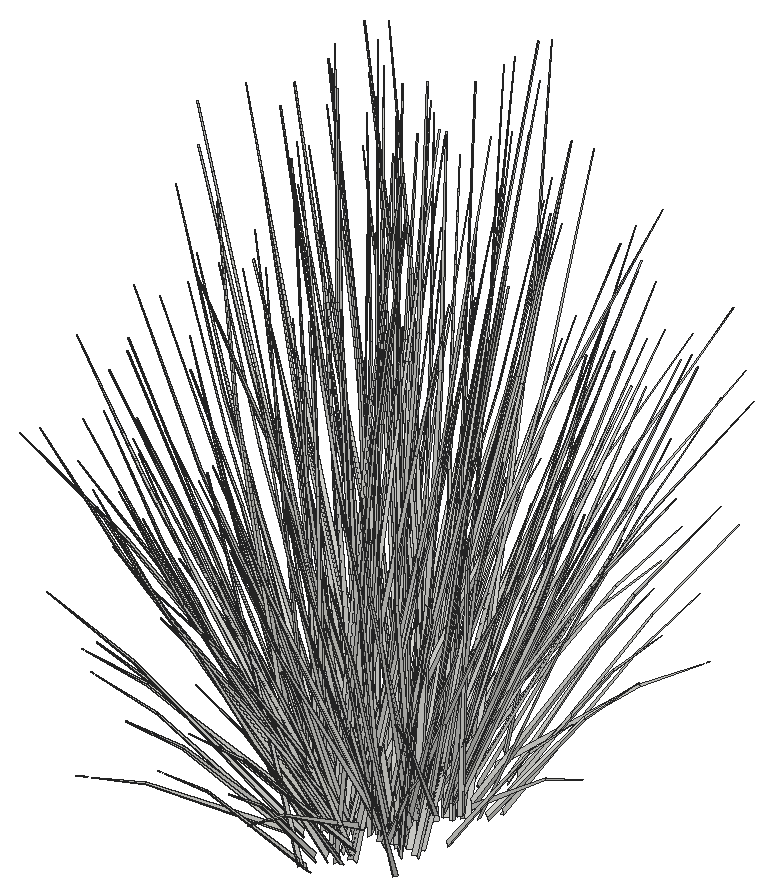
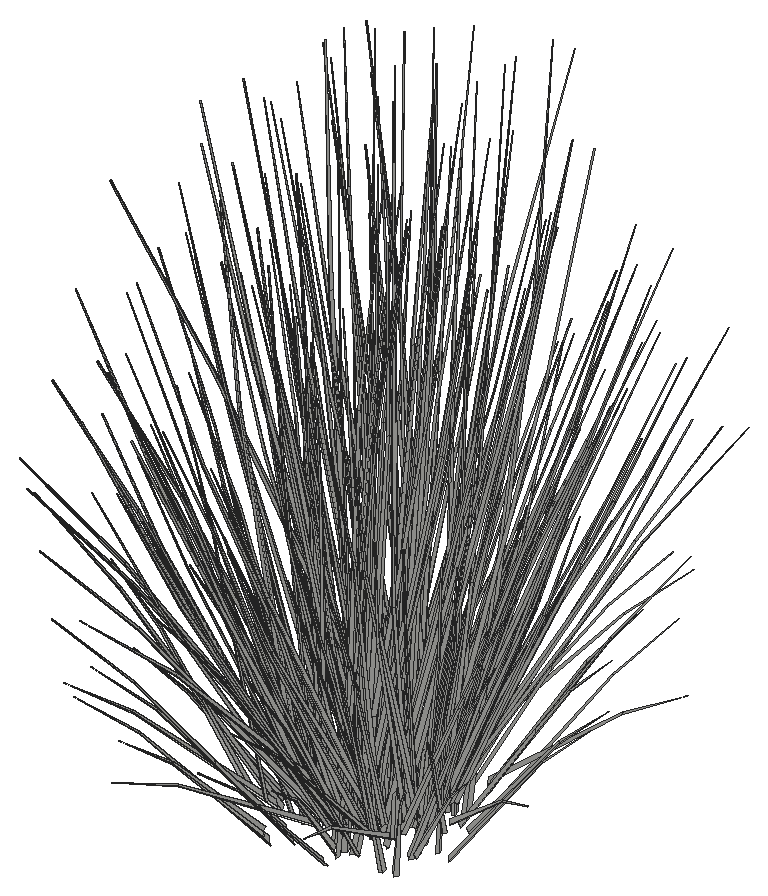
# SketchUp Ruby script. Lengths in inches.
U = 1.inch
M = Sketchup.active_model
def pt(a) = Geom::Point3d.new(a.map { |v| v * U })
def face(e, loops, mat)
  f = e.add_face(loops[0].map { |a| pt(a) })
  loops[1..].each { |l| e.add_face(l.map { |a| pt(a) }).erase! }
  f.material = f.back_material = mat if mat
  f
end
# faces: each face lists its corners as indices into pts; further lists are holes
def faces(e, pts, list, mat = nil) = list.each { |f| face(e, (f[0].is_a?(Array) ? f : [f]).map { |l| l.map { |i| pts[i] } }, mat) }
# xy, xz, yz: faces in a plane at the given z, y or x. An outline is a flat list of corners, or four numbers for a rectangle; further outlines are holes
def ring(l) = l.size == 4 ? [[l[0], l[1]], [l[2], l[1]], [l[2], l[3]], [l[0], l[3]]] : l.each_slice(2).to_a
def flat(e, list, mat, &to3) = list.each { |f| face(e, (f[0].is_a?(Array) ? f : [f]).map { |l| ring(l).map { |u, v| to3.(u, v) } }, mat) }
def xy(e, z, list, mat = nil) = flat(e, list, mat) { |x, y| [x, y, z] }
def xz(e, y, list, mat = nil) = flat(e, list, mat) { |x, z| [x, y, z] }
def yz(e, x, list, mat = nil) = flat(e, list, mat) { |y, z| [x, y, z] }
def lines(e, pts, list) = list.each { |a, b| e.add_line(pt(pts[a]), pt(pts[b])) }
# prism: a flat outline (further loops are holes) pulled along v
def prism(e, loops, v, mat = nil)
  f = face(e, loops, mat); d = Geom::Vector3d.new(v.map { |x| x * U })
  f.pushpull(f.normal.samedirection?(d) ? d.length : -d.length)
end
def box(e, o, s, mat = nil) = prism(e, [[o, [o[0] + s[0], o[1], o[2]], [o[0] + s[0], o[1] + s[1], o[2]], [o[0], o[1] + s[1], o[2]]]], [0, 0, s[2]], mat)
def at(x, y, z, deg = 0) = Geom::Transformation.translation(pt([x, y, z])) * Geom::Transformation.rotation(ORIGIN, Z_AXIS, deg.degrees)
def axes(o, x, y, z) = Geom::Transformation.new([*x, 0, *y, 0, *z, 0, *pt(o).to_a, 1])
def part(name) = M.definitions.add(name)
# library, detail: a bought-in or finely detailed component or shape, given as its bounding box
def library(name, o, s) = part(name).tap { |d| box(d.entities, o, s) }
def detail(e, o, s) = box(e.add_group.entities, o, s)
def put(e, d, t, mat = nil) = e.add_instance(d, t).tap { |i| i.material = mat if mat }
def group(e, t, mat = nil) = e.add_group.tap { |g| g.transformation = t; g.material = mat if mat }.entities
root = M.entities
c1 = part("blade")
p = [[2.15,0.21,22],[0,0.17,0],[0.09,0.45,0],[2.18,0.31,22],[2.29,0.31,22],[0.38,0.45,0],
  [2.48,0.24,33],[2.49,0.24,33],[2.48,0.22,33]]
faces(c1.entities,p,[[0,1,2,3],[4,5,2,3],[6,3,4,7],[8,0,3,6]])
c2 = part("blade with seeds\#1")
put(c2.entities,c1,at(0,0,0))
put(root,c2,axes([454.15,171.57,262.65],[-1.0019,0.47479,-0.62955],[-0.36083,-1.36768,-0.16523],[-0.33927,0.05248,1.38963]))
put(root,c2,axes([455.85,167.23,262.64],[0.89455,-0.42392,-0.62393],[0.32217,1.22114,-0.16376],[0.30292,-0.04686,1.37722]))
put(root,c2,axes([453.97,167.35,262.61],[0.16018,-1.20264,-0.5621],[0.98808,0.25378,-0.14753],[0.11973,-0.3589,1.24074]))
put(root,c2,axes([456.02,171.39,262.61],[-0.16018,1.20264,-0.5621],[-0.98808,-0.25378,-0.14753],[-0.11973,0.3589,1.24074]))
put(root,c2,axes([453.12,169.49,262.61],[-0.73437,-0.77871,-0.5621],[0.66591,-0.96736,-0.14753],[-0.18319,-0.31204,1.24074]))
put(root,c2,axes([456.87,169.25,262.61],[0.73437,0.77871,-0.5621],[-0.66591,0.96736,-0.14753],[0.18319,0.31204,1.24074]))
put(root,c2,axes([452.1,165.78,262.57],[0.48852,-1.08202,-0.44759],[0.87598,0.64674,0],[0.11126,-0.24644,1.41987]))
put(root,c2,axes([458.875,167.96,262.57],[0.48852,1.08202,-0.44759],[-0.87598,0.64674,0],[0.11126,0.24644,1.41987]))
put(root,c2,axes([454.01,174.37,262.57],[-0.97703,0,-0.44759],[0,-1.29348,0],[-0.22253,0,1.41987]))
put(root,c2,axes([457.89,172.96,262.57],[-0.48852,1.08202,-0.44759],[-0.87598,-0.64674,0],[-0.11126,0.24644,1.41987]))
put(root,c2,axes([451.11,170.78,262.57],[-0.48852,-1.08202,-0.44759],[0.87598,-0.64674,0],[-0.11126,-0.24644,1.41987]))
put(root,c2,axes([455.98,164.37,262.57],[0.97703,0,-0.44759],[0,1.29348,0],[0.22253,0,1.41987]))
put(root,c2,axes([454.41,170.85,262.75],[-0.88038,-0.56093,-0.40331],[0.4237,-1.16553,0.1941],[-0.20294,0,1.29492]))
put(root,c2,axes([455.7,170.76,262.75],[-0.82007,0.69452,-0.40331],[-0.57748,-1.05199,0.1941],[-0.10147,0.22475,1.29492]))
put(root,c2,axes([454.29,167.98,262.75],[0.82007,-0.69452,-0.40331],[0.57748,1.05199,0.1941],[0.10147,-0.22475,1.29492]))
put(root,c2,axes([455.58,167.89,262.75],[0.88038,0.56093,-0.40331],[-0.4237,1.16553,0.1941],[0.20294,0,1.29492]))
put(root,c2,axes([456.29,169.28,262.75],[0.06031,1.25545,-0.40331],[-1.00118,0.11354,0.1941],[0.10147,0.22475,1.29492]))
put(root,c2,axes([451.5,170.52,262.58],[0.24175,-1.0786,-0.27926],[0.85134,0.27158,0.27926],[-0.09817,-0.21744,1.25283]))
put(root,c2,axes([455.96,164.92,262.58],[0.60959,0.80703,-0.27926],[-0.60959,0.80703,0.27926],[0.19635,0,1.25283]))
put(root,c2,axes([457.52,172.66,262.58],[-0.85134,0.27158,-0.27926],[-0.24175,-1.0786,0.27926],[-0.09817,0.21744,1.25283]))
put(root,c2,axes([458.49,168.22,262.58],[-0.24175,1.0786,-0.27926],[-0.85134,-0.27158,0.27926],[0.09817,0.21744,1.25283]))
put(root,c2,axes([452.47,166.08,262.58],[0.85134,-0.27158,-0.27926],[0.24175,1.0786,0.27926],[0.09817,-0.21744,1.25283]))
put(root,c2,axes([454.03,173.81,262.58],[-0.60959,-0.80703,-0.27926],[0.60959,-0.80703,0.27926],[-0.19635,0,1.25283]))
put(root,c2,axes([459.05,165.83,262.1],[-0.14106,-0.08423,1.5897],[-0.41543,-1.06044,-0.24285],[0.21501,-0.3215,0.27078]))
put(root,c2,axes([454.62,175.25,262.1],[0.15398,-0.02932,1.5897],[0.80412,0.59108,-0.24285],[-0.04053,0.41985,0.27078]))
put(root,c2,axes([449.4,169.97,262.1],[0.0352,0.19392,1.5897],[-0.39624,1.07238,-0.24285],[-0.33051,-0.01799,0.27078]))
put(root,c2,axes([459.02,170.78,262.1],[-0.05317,-0.18711,1.5897],[0.29263,-1.12549,-0.24285],[0.32981,-0.03291,0.27078]))
put(root,c2,axes([454.77,162.78,262.1],[-0.14833,0.06042,1.5897],[-0.86768,-0.41907,-0.24285],[-0.01248,-0.42273,0.27078]))
put(root,c2,axes([450.61,173.4375,262.1],[0.12871,0.11199,1.5897],[0.2775,1.13173,-0.24285],[-0.25244,0.2734,0.27078]))
put(root,c2,axes([458.93,175.57,262.1],[0.09761,-0.15508,1.5897],[0.90442,-0.26295,-0.24285],[0.19286,0.3437,0.27078]))
put(root,c2,axes([451.09,165.22,262.1],[-0.07697,0.17304,1.5897],[-0.85991,0.44448,-0.24285],[-0.23336,-0.29985,0.27078]))
put(root,c2,axes([453.25,171.66,262.19],[0.39117,1.13797,1.16227],[-1.12236,0.3622,0.45161],[0.01867,-0.69878,1.32195]))
put(root,c2,axes([457.125,168,262.72],[-0.33151,-1.21377,-0.17307],[0.95493,-0.4265,0.00007],[-0.03664,-0.13398,1.56765]))
put(root,c2,axes([456.02,168.4,263.16],[1.11485,-0.13472,-0.26229],[0.06741,1.40314,-0.45076],[0.1485,0.24708,1.43974]))
put(root,c2,axes([454.85,167.75,263.16],[0.46619,-1.302,-0.26229],[0.98396,0.62692,-0.45076],[0.24158,-0.04092,1.43974]))
put(root,c2,axes([455.14,170.99,263.16],[-0.46619,1.302,-0.26229],[-0.98396,-0.62692,-0.45076],[-0.24158,0.04092,1.43974]))
put(root,c2,axes([453.97,170.34,263.16],[-1.11485,0.13472,-0.26229],[-0.06741,-1.40314,-0.45076],[-0.1485,-0.24708,1.43974]))
put(root,c2,axes([453.83,168.72,263.16],[-0.64866,-1.16728,-0.26229],[0.91655,-0.77622,-0.45076],[0.09308,-0.288,1.43974]))
put(root,c2,axes([456.16,170.02,263.16],[0.64866,1.16728,-0.26229],[-0.91655,0.77622,-0.45076],[-0.09308,0.288,1.43974]))
put(root,c2,axes([456.46,168.71,262.98],[-0.78639,1.12892,-0.2271],[-0.88305,-0.94994,0.49699],[0.09199,0.304,1.51643]))
put(root,c2,axes([456.17,170.66,262.95],[-1.15773,-0.30643,-0.21121],[0.20181,-1.4529,0.4622],[-0.15988,0.25387,1.41028]))
put(root,c2,axes([450.09,170.17,262.67],[0.56051,0.79893,-0.03509],[-0.61388,0.73204,-0.15911],[-0.17394,0.05154,0.52479]))
put(root,c2,axes([451.11,174.14,262.67],[0.7978,0.33351,-0.03509],[-0.24541,1.02647,-0.15911],[-0.13049,0.15585,0.52479]))
put(root,c2,axes([454.56,162.23,262.79],[-0.62476,0.71677,-0.05849],[-0.57245,-0.78502,-0.26518],[-0.0403,-0.22243,0.87466]))
put(root,c2,axes([455.38,163.59,262.54],[0.11725,0.74462,1.27635],[-0.9333,0.11852,0.07306],[-0.14126,-0.52153,0.72629]))
put(root,c2,axes([451.27,171.76,262.89],[-0.97904,0.72283,0],[-0.54599,-1.20931,-0.46523],[-0.12435,-0.27543,1.47583]))
put(root,c2,axes([458.48,172.3,262.89],[0.97904,0.72283,0],[-0.54599,1.20931,-0.46523],[-0.12435,0.27543,1.47583]))
put(root,c2,axes([458.72,166.98,262.89],[0.97904,-0.72283,0],[0.54599,1.20931,-0.46523],[0.12435,0.27543,1.47583]))
put(root,c2,axes([454.75,174.69,262.89],[0,1.44565,0],[-1.09198,0,-0.46523],[-0.24871,0,1.47583]))
put(root,c2,axes([457.27,168.77,262.82],[1.12244,-0.50265,-0.0542],[0.39331,1.43622,0],[0.0392,-0.01755,1.55211]))
put(root,c2,axes([451.51,166.43,262.9],[-0.97904,-0.72283,0],[0.54599,-1.20931,-0.46523],[0.12435,-0.27543,1.47583]))
put(root,c2,axes([455.24,164.05,262.9],[0,-1.44565,0],[1.09198,0,-0.46523],[0.24871,0,1.47583]))
put(root,c2,axes([455.51,168.45,262.82],[-0.84094,1.07538,-0.05527],[-0.84146,-1.07603,0],[-0.02937,0.03755,1.58274]))
put(root,c2,axes([455.09,168.08,262.82],[1.12994,0,-0.05082],[0,1.44565,0],[0.03551,0,1.61697]))
put(root,c2,axes([458.61,167.89,262.73],[-0.98246,0.71382,-0.04636],[-0.54599,-1.20931,0.46523],[0.09354,0.298,1.4751]))
put(root,c2,axes([455.8,164.62,262.74],[-0.00781,1.44494,-0.04486],[-1.09198,0,0.45022],[0.24858,0.04541,1.42752]))
put(root,c2,axes([454.46,173.57,262.85],[0.82143,1.07538,0.27726],[-0.81279,1.07603,-0.32897],[-0.23327,0.03755,1.48641]))
put(root,c2,axes([458.11,167.86,262.85],[0.31757,-1.44738,0.27726],[1.13512,0.3621,-0.32897],[0.14207,0.23956,1.48641]))
put(root,c2,axes([457.625,169.68,262.73],[-0.43865,1.16553,0],[-0.91144,-0.56093,0],[0,0,1.46678]))
put(root,c2,axes([457.24,169.41,262.74],[-0.84234,0.37722,0],[-0.29498,-1.07717,0],[0,0,1.39163]))
put(root,c2,axes([457.64,168.35,262.74],[0.43865,-1.16553,0],[0.91144,0.56093,0],[0,0,1.57718]))
put(root,c2,axes([454.64,168.81,262.74],[-1.1305,0,0],[0,-1.44565,0],[0,0,1.61777]))
put(root,c2,axes([454.89,167.83,262.74],[0,-1.29348,0],[1.0115,0,0],[0,0,1.60831]))
put(root,c2,axes([455.32,167.86,262.75],[0.63109,-0.80703,0],[0.63109,0.80703,0],[0,0,1.52591]))
put(root,c2,axes([455.61,170.49,262.88],[0.20585,-1.46124,0.41247],[1.16261,0.29738,0.16186],[-0.11226,0.21355,1.43206]))
put(root,c2,axes([453.92,169.49,262.88],[0.88667,0.95859,0.41247],[-0.7827,1.13884,0.16186],[-0.08849,-0.2311,1.43206]))
put(root,c2,axes([454.54,170.62,262.88],[1.09253,-0.50265,0.41247],[0.37991,1.43622,0.16186],[-0.20075,-0.01755,1.43206]))
put(root,c2,axes([454.375,168.25,262.9],[-0.20585,1.46124,0.44352],[-1.16261,-0.29738,0.17404],[0.11226,-0.21355,1.53985]))
put(root,c2,axes([456.24,168.14,263.11],[0.58702,-0.85413,0.13053],[0.66228,0.71246,-0.37274],[0.08953,0.19831,1.14258]))
put(root,c2,axes([453.54,168.61,263.11],[-0.87196,-0.22303,0.13053],[0.15136,-1.08968,-0.37274],[0.08953,-0.19831,1.14258]))
put(root,c2,axes([454.79,167.38,263.11],[-0.28493,-1.07717,0.13053],[0.81364,-0.37722,-0.37274],[0.17907,0,1.14258]))
put(root,c2,axes([456.45,170.13,263.11],[0.87196,0.22303,0.13053],[-0.15136,1.08968,-0.37274],[-0.08953,0.19831,1.14258]))
put(root,c2,axes([459.15,173.37,263.3],[-0.17302,-1.05027,0.05866],[0.69705,-0.24145,-0.77802],[0.35285,0.06658,0.69739]))
put(root,c2,axes([452.8,174.45,263.09],[0.27202,-0.22572,1.28914],[0.7394,0.52014,-0.27724],[-0.17673,0.53408,0.55117]))
put(root,c2,axes([459.89,173.62,263.09],[-0.15413,-0.36483,1.28914],[0.46474,-0.90077,-0.27724],[0.40213,0.2681,0.55117]))
put(root,c2,axes([457.71,168.33,263.09],[-0.32388,-0.0204,1.28914],[-0.36177,-0.97496,-0.27724],[0.38765,-0.30097,0.55117]))
put(root,c2,axes([450.47,167.52,263.09],[0.19776,0.32863,1.28914],[-0.34614,0.98419,-0.27724],[-0.43048,-0.18244,0.55117]))
put(root,c2,axes([452.8,164.35,263.09],[-0.02894,0.41302,1.28914],[-0.77632,0.42312,-0.27724],[-0.21961,-0.50739,0.55117]))
put(root,c2,axes([450.1,172.61,263.09],[0.31962,0.07001,1.28914],[0.26756,1.02347,-0.27724],[-0.41311,0.23924,0.55117]))
put(root,c2,axes([456.77,163.38,263.09],[-0.2403,0.27843,1.28914],[-0.79492,-0.36227,-0.27724],[0.10768,-0.56334,0.55117]))
put(root,c2,axes([456.76,176,263.09],[0.08021,-0.40179,1.28914],[0.81924,-0.25896,-0.27724],[0.15335,0.54576,0.55117]))
put(root,c2,axes([454.91,173.81,262.99],[0.97703,0,0.44759],[0,1.29348,0],[-0.22253,0,1.41987]))
put(root,c2,axes([452.02,167.06,262.99],[-0.48852,1.08202,0.44759],[-0.87598,-0.64674,0],[0.11126,-0.24644,1.41987]))
put(root,c2,axes([455.08,164.92,262.99],[-0.97703,0,0.44759],[0,-1.29348,0],[0.22253,0,1.41987]))
put(root,c2,axes([458.05,167.24,262.99],[-0.48852,-1.08202,0.44759],[0.87598,-0.64674,0],[0.11126,0.24644,1.41987]))
put(root,c2,axes([457.97,171.68,262.99],[0.48852,-1.08202,0.44759],[0.87598,0.64674,0],[-0.11126,0.24644,1.41987]))
put(root,c2,axes([454.84,170.15,262.95],[0.47355,-1.30265,0.21694],[0.98396,0.62692,0.45076],[-0.22682,0,1.44726]))
put(root,c2,axes([452.52,167.46,262.98],[0.25932,1.24233,0.15904],[-0.96507,0.30677,0.3163],[0.14061,-0.1108,1.44604]))
put(root,c2,axes([455.05,165.67,262.98],[-0.71168,0.90835,0.15904],[-0.69029,-0.91538,0.3163],[0.14534,0.10032,1.44604]))
put(root,c2,axes([452.46,171.16,262.98],[0.971,0.33398,0.15904],[-0.27478,1.22215,0.3163],[-0.00473,-0.21112,1.44604]))
put(root,c2,axes([457.53,167.58,262.98],[-0.971,-0.33398,0.15904],[0.27478,-1.22215,0.3163],[0.00473,0.21112,1.44604]))
put(root,c2,axes([457.47,171.28,262.98],[-0.25932,-1.24233,0.15904],[0.96507,-0.30677,0.3163],[-0.14061,0.1108,1.44604]))
put(root,c2,axes([454.58,167.87,263.2],[-0.88038,-0.56093,0.40331],[0.4237,-1.16553,-0.1941],[0.20294,0,1.29492]))
put(root,c2,axes([454.18,170.57,263.2],[0.06031,1.25545,0.40331],[-1.00118,0.11354,-0.1941],[-0.10147,-0.22475,1.29492]))
put(root,c2,axes([453.77,169.07,263.2],[-0.82007,0.69452,0.40331],[-0.57748,-1.05199,-0.1941],[0.10147,-0.22475,1.29492]))
put(root,c2,axes([455.4,170.87,263.2],[0.88038,0.56093,0.40331],[-0.4237,1.16553,-0.1941],[-0.20294,0,1.29492]))
put(root,c2,axes([455.81,168.16,263.2],[-0.06031,-1.25545,0.40331],[1.00118,-0.11354,-0.1941],[0.10147,0.22475,1.29492]))
put(root,c2,axes([459.29,165.91,263.16],[-0.03064,0.74138,0.9471],[-0.6508,-0.48961,0.52291],[0.23122,-0.29288,0.74292]))
put(root,c2,axes([453.61,175.79,263.25],[-0.06991,-0.73811,1.03545],[0.616,0.4682,0.76078],[-0.09241,0.36475,0.22807]))
put(root,c2,axes([458.01,166.01,263.25],[-0.28093,0.65095,1.03545],[-0.28545,-0.84053,0.76078],[0.2418,-0.22671,0.22807]))
put(root,c2,axes([458.48,176.84,263.25],[-0.44281,-0.48182,1.03545],[0.70101,-0.19012,0.76078],[0.12552,0.34819,0.22807]))
put(root,c2,axes([455.7,162.04,263.25],[0.1613,0.71432,1.03545],[-0.66662,-0.33623,0.76078],[0.04561,-0.37895,0.22807]))
put(root,c2,axes([449.59,172.96,263.25],[0.34005,-0.60308,1.03545],[0.20441,0.87829,0.76078],[-0.26134,0.18792,0.22807]))
put(root,c2,axes([460.41,172.75,263.25],[-0.58095,0.02992,1.03545],[0.41436,-0.74764,0.76078],[0.2769,0.14704,0.22807]))
put(root,c2,axes([451.375,163.88,263.25],[0.49736,0.38508,1.03545],[-0.66822,0.331,0.76078],[-0.16744,-0.31805,0.22807]))
put(root,c2,axes([448.9,168.73,263.25],[0.56973,-0.14831,1.03545],[-0.31555,0.82274,0.76078],[-0.29172,-0.08853,0.22807]))
put(root,c2,axes([454.85,167.6,263.32],[-0.91991,0.03158,1.27354],[0.23846,-1.42935,0.53923],[0.50337,0.33806,1.20213]))
put(root,c2,axes([451.39,171.51,265.24],[-0.47225,0.98582,-0.64046],[-0.82754,-0.7006,0.07729],[-0.28197,0.35717,0.906]))
put(root,c2,axes([458.64,170.43,265.24],[0.79444,-0.5518,-0.64046],[0.44274,1.13586,0.07729],[0.38385,-0.12903,0.906]))
put(root,c2,axes([452.56,173.51,265.24],[-0.02352,1.1557,-0.64046],[-0.99061,-0.07762,0.07729],[-0.10454,0.48961,0.906]))
put(root,c2,axes([453.51,165.23,265.24],[-0.77091,-0.6039,-0.64046],[0.54787,-1.05824,0.07729],[-0.27931,-0.36058,0.906]))
put(root,c2,axes([455.46,164.94,265.24],[-0.4315,-1.0159,-0.64046],[0.88824,-0.56616,0.07729],[-0.1009,-0.49086,0.906]))
put(root,c2,axes([451.94,166.72,265.24],[-0.90375,-0.03008,-0.64046],[0.0607,-1.26677,0.07729],[-0.38287,-0.13368,0.906]))
put(root,c2,axes([457.25,165.93,265.24],[0.02352,-1.1557,-0.64046],[0.99061,0.07762,0.07729],[0.10454,-0.48961,0.906]))
put(root,c2,axes([451.16,169.02,265.24],[-0.79444,0.5518,-0.64046],[-0.44274,-1.13586,0.07729],[-0.38385,0.12903,0.906]))
put(root,c2,axes([458.8,170.02,264.97],[0.24493,-1.13649,-0.46065],[0.83975,0.38955,-0.35681],[0.33809,-0.10421,0.88141]))
put(root,c2,axes([451.64,166.98,264.97],[-0.65648,0.82762,-0.46065],[-0.57493,-0.87428,-0.35681],[-0.33354,-0.12593,0.88141]))
put(root,c2,axes([451.41,171.97,264.97],[0.23225,1.14083,-0.46065],[-0.87956,0.19957,-0.35681],[-0.25205,0.30642,0.88141]))
put(root,c2,axes([455.13,164.74,264.97],[-0.88873,-0.31321,-0.46065],[0.30463,-1.07385,-0.35681],[-0.08149,-0.43235,0.88141]))
put(root,c2,axes([452.76,173.9,264.97],[0.6472,0.83949,-0.46065],[-0.68369,0.73521,-0.35681],[-0.09847,0.42653,0.88141]))
put(root,c2,axes([456.66,174.19,264.97],[0.89213,-0.297,-0.46065],[0.15606,1.12475,-0.35681],[0.23962,0.32232,0.88141]))
put(root,c2,axes([454.68,174.71,264.97],[0.88873,0.31321,-0.46065],[-0.30463,1.07385,-0.35681],[0.08149,0.43235,0.88141]))
put(root,c2,axes([451,169.43,264.97],[-0.24493,1.13649,-0.46065],[-0.83975,-0.38955,-0.35681],[-0.33809,0.10421,0.88141]))
put(root,c2,axes([453.15,165.26,264.97],[-0.89213,0.297,-0.46065],[-0.15606,-1.12475,-0.35681],[-0.23962,-0.32232,0.88141]))
put(root,c2,axes([458.4,167.48,264.97],[-0.23225,-1.14083,-0.46065],[0.87956,-0.19957,-0.35681],[0.25205,-0.30642,0.88141]))
put(root,c2,axes([454.14,172.44,263.77],[-0.14134,-0.32863,1.5962],[0.98684,-0.11332,0.12492],[0.13095,0.71181,0.57049]))
put(root,c2,axes([457.87,172.73,265.57],[0.90375,0.03008,-0.71091],[-0.0607,1.26677,0.08579],[0.38287,0.13368,1.00565]))
put(root,c2,axes([458.17,172.47,265.27],[0.65648,-0.82762,-0.51132],[0.57493,0.87428,-0.39606],[0.33354,0.12593,0.97836]))
put(root,c2,axes([459.14,173.15,263.79],[-0.50438,-0.0254,1.3914],[0.26641,-1.14247,0.19228],[0.53755,0.09899,0.65702]))
put(root,c2,axes([456.73,169.15,263.75],[0.39398,-0.99907,1.36359],[0.84877,0.97875,0.53923],[-0.50305,0.4384,1.14314]))
put(root,c2,axes([457.66,165.24,264.83],[0.61172,-0.65782,-0.31925],[0.57907,0.75112,0.41216],[0.08811,-0.38163,0.78863]))
put(root,c2,axes([454.27,175.37,264.83],[-0.27256,0.96081,-0.31925],[-0.79518,-0.28024,0.41216],[0.07291,0.38684,0.78863]))
put(root,c2,axes([456.5625,175.02,264.83],[0.13963,1.00636,-0.31925],[-0.79822,0.26574,0.41216],[0.2144,0.28839,0.78863]))
put(root,c2,axes([455.54,164.08,264.83],[0.27256,-0.96081,-0.31925],[0.79518,0.28024,0.41216],[-0.07291,-0.38684,0.78863]))
put(root,c2,axes([450.76,171.85,264.83],[-0.78697,0.17856,-0.31925],[-0.2078,-1.02074,0.41216],[-0.22552,0.27417,0.78863]))
put(root,c2,axes([458.41,173.25,264.83],[0.51441,0.78225,-0.31925],[-0.58738,0.7405,0.41216],[0.29843,0.11267,0.78863]))
put(root,c2,axes([453.24,164.43,264.83],[-0.13963,-1.00636,-0.31925],[0.79822,-0.26574,0.41216],[-0.2144,-0.28839,0.78863]))
put(root,c2,axes([459.32,170.53,264.83],[0.75135,0.34854,-0.31925],[-0.21915,1.01686,0.41216],[0.30251,-0.09324,0.78863]))
put(root,c2,axes([451.4,166.2,264.83],[-0.51441,-0.78225,-0.31925],[0.58738,-0.7405,0.41216],[-0.29843,-0.11267,0.78863]))
put(root,c2,axes([450.49,168.91,264.83],[-0.75135,-0.34854,-0.31925],[0.21915,-1.01686,0.41216],[-0.30251,0.09324,0.78863]))
put(root,c2,axes([452.15,174.21,264.83],[-0.61172,0.65782,-0.31925],[-0.57907,-0.75112,0.41216],[-0.08811,0.38163,0.78863]))
put(root,c2,axes([457.75,163.28,264.3],[-0.82131,0.22128,-0.03148],[-0.18882,-1.04586,-0.14272],[0.05207,-0.2184,0.47074]))
put(root,c2,axes([456.09,167.6,264.25],[-0.16834,0.42944,1.54493],[-0.70619,-0.88871,0.12492],[0.31858,-0.5539,0.66044]))
put(root,c2,axes([451.48,168.15,264.25],[0.33582,0.21526,1.54493],[-0.69497,0.90306,0.12492],[-0.43315,-0.40739,0.66044]))
put(root,c2,axes([454.55,166.7,264.25],[0.02213,0.47954,1.54493],[-0.95907,-0.31812,0.12492],[0.05932,-0.68338,0.66044]))
put(root,c2,axes([457.07,169.37,264.25],[-0.31369,0.26428,1.54493],[-0.26409,-1.22118,0.12492],[0.49247,-0.276,0.66044]))
put(root,c2,axes([457.23,171.53,264.25],[-0.375,0.0283,1.54493],[0.24877,-1.22643,0.12492],[0.53441,0.07586,0.66044]))
put(root,c2,axes([456.52,173.5,264.25],[-0.33582,-0.21526,1.54493],[0.69497,-0.90306,0.12492],[0.43315,0.40739,0.66044]))
put(root,c2,axes([455.13,174.75,264.25],[-0.20666,-0.40114,1.54493],[0.95496,-0.33772,0.12492],[0.21583,0.62976,0.66044]))
put(root,c2,axes([455.78,173.28,264.25],[-0.3002,-0.28876,1.54493],[0.81031,-0.72911,0.12492],[0.36902,0.50009,0.66044]))
put(root,c2,axes([450.93,172.27,264.25],[0.31369,-0.26428,1.54493],[0.26409,1.22118,0.12492],[-0.49247,0.276,0.66044]))
put(root,c2,axes([451.91,174.04,264.25],[0.16834,-0.42944,1.54493],[0.70619,0.88871,0.12492],[-0.31858,0.5539,0.66044]))
put(root,c2,axes([453.45,174.95,264.25],[-0.02213,-0.47954,1.54493],[0.95907,0.31812,0.12492],[-0.05932,0.68338,0.66044]))
put(root,c2,axes([457.73,165.99,265.29],[-0.99362,-0.0619,-0.10962],[0.02716,-1.17208,-0.60845],[0.06902,-0.45141,0.92453]))
put(root,c2,axes([453.92,174.76,265.29],[0.88471,-0.5817,-0.10962],[0.43476,1.03242,-0.60845],[0.11673,0.43507,0.92453]))
put(root,c2,axes([451.98,166.11,265.29],[-0.04841,1.27062,-0.10962],[-0.91657,-0.03473,-0.60845],[-0.353,-0.08826,0.92453]))
put(root,c2,axes([455.89,164.68,265.29],[-0.88471,0.5817,-0.10962],[-0.43476,-1.03242,-0.60845],[-0.11673,-0.43507,0.92453]))
put(root,c2,axes([458.84,170.99,265.29],[-0.45489,-1.13134,-0.10962],[0.80735,-0.55596,-0.60845],[0.34022,-0.14927,0.92453]))
put(root,c2,axes([452.08,173.46,265.29],[0.99362,0.0619,-0.10962],[-0.02716,1.17208,-0.60845],[-0.06902,0.45141,0.92453]))
put(root,c2,axes([458.81,168.3,265.29],[-0.8363,-0.68892,-0.10962],[0.4818,-0.99769,-0.60845],[0.23628,-0.3468,0.92453]))
put(root,c2,axes([456.02,174.72,265.29],[0.53874,-1.06944,-0.10962],[0.78019,0.61612,-0.60845],[0.2712,0.30214,0.92453]))
put(root,c2,axes([450.96,168.46,265.29],[0.45489,1.13134,-0.10962],[-0.80735,0.55596,-0.60845],[-0.34022,0.14927,0.92453]))
put(root,c2,axes([453.79,164.73,265.29],[-0.53874,1.06944,-0.10962],[-0.78019,-0.61612,-0.60845],[-0.2712,-0.30214,0.92453]))
put(root,c2,axes([453.875,167.52,264.79],[-0.50765,0.99901,1.24659],[-0.79039,-1.05487,0.53787],[0.47632,-0.32232,1.20495]))
put(root,c2,axes([454.8,175.98,265],[0.12685,0.18879,1.57709],[0.92682,-0.01606,-0.24942],[0.12053,0.43275,0.12648]))
put(root,c2,axes([454.5,161.53,265],[-0.14882,-0.16043,1.57709],[-0.91289,0.20534,-0.24942],[-0.17308,-0.40254,0.12648]))
put(root,c2,axes([457.13,164.97,265],[-0.01652,-0.24801,1.57709],[-0.75906,-0.68026,-0.24942],[0.1002,-0.44114,0.12648]))
put(root,c2,axes([450.53,164.96,265],[-0.19445,0.01116,1.57709],[-0.562,0.94258,-0.24942],[-0.34067,-0.14573,0.12648]))
put(root,c2,axes([458.26,175.95,265],[0.19335,0.02874,1.57709],[0.67262,-0.81555,-0.24942],[0.31807,0.21351,0.12648]))
put(root,c2,axes([460.65,171.25,265],[0.15733,-0.14655,1.57709],[0.06181,-1.18266,-0.24942],[0.34698,-0.11893,0.12648]))
put(root,c2,axes([448.85,170.26,265],[-0.13699,0.17683,1.57709],[0.08685,1.18009,-0.24942],[-0.32765,0.18834,0.12648]))
put(root,c2,axes([450.36,174.125,265],[-0.0069,0.24875,1.57709],[0.68965,0.79195,-0.24942],[-0.14092,0.42256,0.12648]))
put(root,c2,axes([450.94,175.08,265],[0.0975,-0.08571,1.59908],[0.87648,0.41319,-0.1511],[0.00634,0.41846,0.28298]))
put(root,c2,axes([448.4,171.47,265],[0.11711,0.02157,1.59908],[0.42502,1.06376,-0.1511],[-0.21726,0.31303,0.28298]))
put(root,c2,axes([459.5,169.2,265],[-0.11829,-0.00342,1.59908],[-0.52187,-0.99076,-0.1511],[0.18628,-0.34414,0.28298]))
put(root,c2,axes([455.74,178.07,265],[0.0262,-0.14755,1.59908],[0.86326,-0.45644,-0.1511],[0.22658,0.30203,0.28298]))
put(root,c2,axes([453.56,162.1,265],[-0.00742,0.151,1.59908],[-0.79509,0.62706,-0.1511],[-0.26143,-0.25182,0.28298]))
put(root,c2,axes([458.52,162.37,265],[-0.08553,0.10454,1.59908],[-0.91687,-0.22868,-0.1511],[-0.05858,-0.41178,0.28298]))
put(root,c2,axes([460.24,176.04,265],[-0.05899,-0.13116,1.59908],[0.39237,-1.08407,-0.1511],[0.32669,0.02548,0.28298]))
put(root,c2,axes([449.83,165.21,265],[0.07463,0.11741,1.59908],[-0.25178,1.15035,-0.1511],[-0.32567,0.04164,0.28298]))
put(root,c2,axes([457.82,173.34,265.62],[0.04841,-1.27062,-0.12168],[0.91657,0.03473,-0.67538],[0.353,0.08826,1.02623]))
put(root,c2,axes([450.625,171.17,265.65],[0.93666,0.77159,-0.12278],[-0.53962,1.11741,-0.68147],[-0.26463,0.38842,1.03548]))
put(root,c2,axes([450.66,168.79,265.02],[0.25543,-1.1392,0.43274],[0.83975,0.38955,0.35681],[-0.33023,0.06846,0.89544]))
put(root,c2,axes([457.66,165.49,265.02],[0.64379,0.85247,0.43274],[-0.68369,0.73521,0.35681],[0.11875,-0.39995,0.89544]))
put(root,c2,axes([455.64,164.3,265.02],[0.89085,0.32663,0.43274],[-0.30463,1.07385,0.35681],[-0.05354,-0.4223,0.89544]))
put(root,c2,axes([456.39,174.89,265.02],[-0.89921,0.28673,0.43274],[-0.15606,-1.12475,0.35681],[0.21148,0.33149,0.89544]))
put(root,c2,axes([458.21,173.25,265.02],[-0.66663,0.82326,0.43274],[-0.57493,-0.87428,0.35681],[0.31276,0.15186,0.89544]))
put(root,c2,axes([451.6,166.2,265.02],[0.66663,-0.82326,0.43274],[0.57493,0.87428,0.35681],[-0.31276,-0.15186,0.89544]))
put(root,c2,axes([454.17,175.15,265.02],[-0.89085,-0.32663,0.43274],[0.30463,-1.07385,0.35681],[0.05354,0.4223,0.89544]))
put(root,c2,axes([453.42,164.56,265.02],[0.89921,-0.28673,0.43274],[0.15606,1.12475,0.35681],[-0.21148,-0.33149,0.89544]))
put(root,c2,axes([458.94,167.82,265.02],[0.22422,1.14989,0.43274],[-0.87956,0.19957,0.35681],[0.25922,-0.27044,0.89544]))
put(root,c2,axes([450.69,171.4,265.02],[-0.62066,-0.52545,0.05797],[0.36135,-0.74826,0.45634],[-0.19899,0.24191,0.69585]))
put(root,c2,axes([459.21,170.96,265.02],[0.33205,0.8519,0.05797],[-0.60551,0.41697,0.45634],[0.26692,-0.08227,0.69585]))
put(root,c2,axes([453.59,164.34,265.02],[0.4109,-0.79368,0.05797],[0.58514,0.46209,0.45634],[-0.18917,-0.25446,0.69585]))
put(root,c2,axes([455.87,164.22,265.02],[0.66618,-0.42462,0.05797],[0.32607,0.77431,0.45634],[-0.06434,-0.34133,0.69585]))
put(root,c2,axes([451.91,173.87,265.02],[-0.74296,-0.05822,0.05797],[0.02037,-0.87906,0.45634],[-0.07774,0.33673,0.69585]))
put(root,c2,axes([451.66,165.9,265.02],[0.04552,-0.95007,0.05797],[0.68742,0.02605,0.45634],[-0.26332,-0.09941,0.69585]))
put(root,c2,axes([457.89,165.58,265.02],[0.74296,0.05822,0.05797],[-0.02037,0.87906,0.45634],[0.07774,-0.33673,0.69585]))
put(root,c2,axes([456.22,175.11,265.02],[-0.4109,0.79368,0.05797],[-0.58514,-0.46209,0.45634],[0.18917,0.25446,0.69585]))
put(root,c2,axes([450.6,168.49,265.02],[-0.33205,-0.8519,0.05797],[0.60551,-0.41697,0.45634],[-0.26692,0.08227,0.69585]))
put(root,c2,axes([453.9375,175.23,265.02],[-0.66618,0.42462,0.05797],[-0.32607,-0.77431,0.45634],[0.06434,0.34133,0.69585]))
put(root,c2,axes([459.12,168.04,265.02],[0.62066,0.52545,0.05797],[-0.36135,0.74826,0.45634],[0.19899,-0.24191,0.69585]))
put(root,c2,axes([458.15,173.55,265.02],[-0.04552,0.95007,0.05797],[-0.68742,-0.02605,0.45634],[0.26332,0.09941,0.69585]))
put(root,c2,axes([458.53,170.65,265.31],[-0.75135,-0.34854,0.31925],[0.21915,-1.01686,-0.41216],[0.30251,-0.09324,0.78863]))
put(root,c2,axes([451.28,168.8,265.31],[0.75135,0.34854,0.31925],[-0.21915,1.01686,-0.41216],[-0.30251,0.09324,0.78863]))
put(root,c2,axes([457.34,166.17,265.31],[-0.61172,0.65782,0.31925],[-0.57907,-0.75112,-0.41216],[0.08811,-0.38163,0.78863]))
put(root,c2,axes([455.625,165.09,265.31],[-0.27256,0.96081,0.31925],[-0.79518,-0.28024,-0.41216],[-0.07291,-0.38684,0.78863]))
put(root,c2,axes([452.47,173.28,265.31],[0.61172,-0.65782,0.31925],[0.57907,0.75112,-0.41216],[-0.08811,0.38163,0.78863]))
put(root,c2,axes([457.68,172.84,265.31],[-0.51441,-0.78225,0.31925],[0.58738,-0.7405,-0.41216],[0.29843,0.11267,0.78863]))
put(root,c2,axes([456.09,174.2,265.31],[-0.13963,-1.00636,0.31925],[0.79822,-0.26574,-0.41216],[0.2144,0.28839,0.78863]))
put(root,c2,axes([458.4,168.21,265.31],[-0.78697,0.17856,0.31925],[-0.2078,-1.02074,-0.41216],[0.22552,-0.27417,0.78863]))
put(root,c2,axes([453.72,165.25,265.31],[0.13963,1.00636,0.31925],[-0.79822,0.26574,-0.41216],[-0.2144,-0.28839,0.78863]))
put(root,c2,axes([454.18,174.36,265.31],[0.27256,-0.96081,0.31925],[0.79518,0.28024,-0.41216],[0.07291,0.38684,0.78863]))
put(root,c2,axes([452.125,166.61,265.31],[0.51441,0.78225,0.31925],[-0.58738,0.7405,-0.41216],[-0.29843,-0.11267,0.78863]))
put(root,c2,axes([451.4,171.24,265.31],[0.78697,-0.17856,0.31925],[0.2078,1.02074,-0.41216],[-0.22552,0.27417,0.78863]))
put(root,c2,axes([459.15,170.66,265.32],[-0.25543,1.1392,0.48034],[-0.83975,-0.38955,0.39606],[0.33023,-0.06846,0.99394]))
put(root,c2,axes([451.92,174.31,265.35],[-0.72104,-0.95477,0.48466],[0.76573,-0.82343,0.39963],[-0.133,0.44794,1.00289]))
put(root,c2,axes([450.48,171.7,265.35],[-0.25113,-1.28788,0.48466],[0.9851,-0.22351,0.39963],[-0.29033,0.30289,1.00289]))
put(root,c2,axes([461.21,169.28,265.84],[-0.56051,-0.79893,-0.05849],[0.61388,-0.73204,-0.26518],[0.17394,-0.05154,0.87466]))
put(root,c2,axes([458.36,176.48,265.84],[0.2608,-1.0202,-0.05849],[0.8027,0.31383,-0.26518],[0.12187,0.16686,0.87466]))
